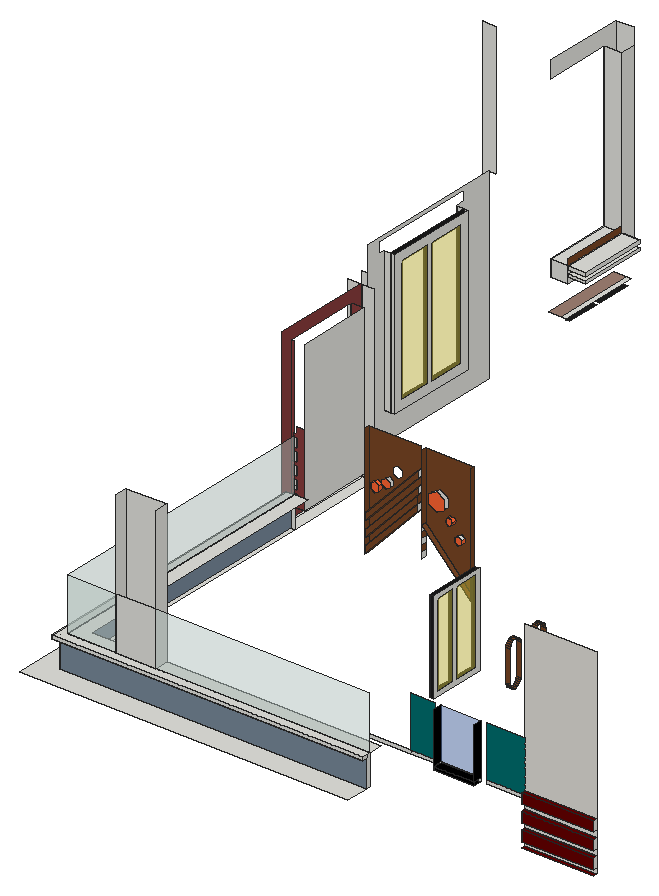
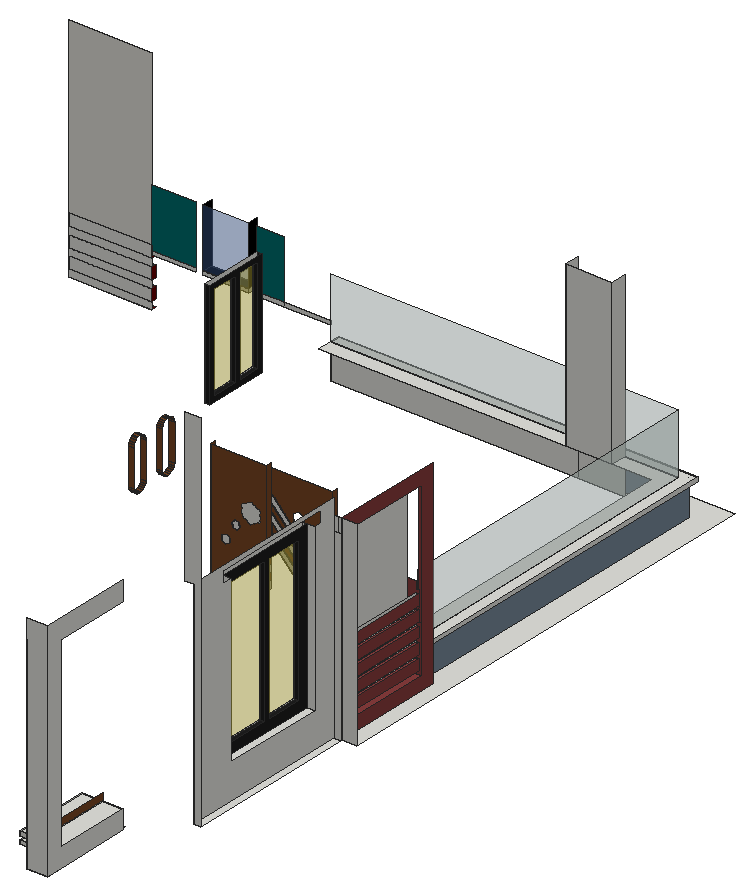
# SketchUp Ruby script. Lengths in inches.
U = 1.inch
M = Sketchup.active_model
def pt(a) = Geom::Point3d.new(a.map { |v| v * U })
def face(e, loops, mat)
  f = e.add_face(loops[0].map { |a| pt(a) })
  loops[1..].each { |l| e.add_face(l.map { |a| pt(a) }).erase! }
  f.material = f.back_material = mat if mat
  f
end
# faces: each face lists its corners as indices into pts; further lists are holes
def faces(e, pts, list, mat = nil) = list.each { |f| face(e, (f[0].is_a?(Array) ? f : [f]).map { |l| l.map { |i| pts[i] } }, mat) }
# xy, xz, yz: faces in a plane at the given z, y or x. An outline is a flat list of corners, or four numbers for a rectangle; further outlines are holes
def ring(l) = l.size == 4 ? [[l[0], l[1]], [l[2], l[1]], [l[2], l[3]], [l[0], l[3]]] : l.each_slice(2).to_a
def flat(e, list, mat, &to3) = list.each { |f| face(e, (f[0].is_a?(Array) ? f : [f]).map { |l| ring(l).map { |u, v| to3.(u, v) } }, mat) }
def xy(e, z, list, mat = nil) = flat(e, list, mat) { |x, y| [x, y, z] }
def xz(e, y, list, mat = nil) = flat(e, list, mat) { |x, z| [x, y, z] }
def yz(e, x, list, mat = nil) = flat(e, list, mat) { |y, z| [x, y, z] }
def lines(e, pts, list) = list.each { |a, b| e.add_line(pt(pts[a]), pt(pts[b])) }
# prism: a flat outline (further loops are holes) pulled along v
def prism(e, loops, v, mat = nil)
  f = face(e, loops, mat); d = Geom::Vector3d.new(v.map { |x| x * U })
  f.pushpull(f.normal.samedirection?(d) ? d.length : -d.length)
end
def box(e, o, s, mat = nil) = prism(e, [[o, [o[0] + s[0], o[1], o[2]], [o[0] + s[0], o[1] + s[1], o[2]], [o[0], o[1] + s[1], o[2]]]], [0, 0, s[2]], mat)
def at(x, y, z, deg = 0) = Geom::Transformation.translation(pt([x, y, z])) * Geom::Transformation.rotation(ORIGIN, Z_AXIS, deg.degrees)
def axes(o, x, y, z) = Geom::Transformation.new([*x, 0, *y, 0, *z, 0, *pt(o).to_a, 1])
def part(name) = M.definitions.add(name)
# library, detail: a bought-in or finely detailed component or shape, given as its bounding box
def library(name, o, s) = part(name).tap { |d| box(d.entities, o, s) }
def detail(e, o, s) = box(e.add_group.entities, o, s)
def put(e, d, t, mat = nil) = e.add_instance(d, t).tap { |i| i.material = mat if mat }
def group(e, t, mat = nil) = e.add_group.tap { |g| g.transformation = t; g.material = mat if mat }.entities
root = M.entities
M.materials.add("Niraj_Skin").color = [158, 128, 115]
M.materials.add("[0017_IndianRed]").color = [135, 60, 60]
M.materials.add("[0110_LightSlateGray]").color = [119, 136, 153]
M.materials.add("[Color A08]").color = [102, 0, 0]
M.materials.add("[Color B04]").color = [255, 101, 50]
M.materials.add("[Color H07]1").color = [0, 109, 109]
M.materials.add("[Color M08]").color = [30, 30, 30]
M.materials.add("[Color M09]").color = [0, 0, 0]
M.materials.add("[Marble Carrara Gold Floor Tile]").color = [225, 223, 217]
M.materials.add("[Translucent Glass Blue]").color = [218, 237, 231]
M.materials["[Translucent Glass Blue]"].alpha = 0.5
M.materials.add("[Translucent Glass Blue]1").color = [78, 117, 186]
M.materials["[Translucent Glass Blue]1"].alpha = 0.5
M.materials.add("[Translucent Glass Gray]").color = [242, 225, 74]
M.materials["[Translucent Glass Gray]"].alpha = 0.5
M.materials.add("[Wood Veneer 01]").color = [120, 70, 37]
xy(root,135.72,[[72.04,94.04,294.79,94.04,294.79,109.91,86.54,109.91,86.54,305.6,80.6,305.6,80.6,372.52,72.04,372.52],[86.54,109.91,121.875,112.91],[121.875,109.91,149.09,112.91],[149.09,109.91,294.79,112.91],[86.54,112.91,89.54,305.6],
  [80.6,305.6,82.23,372.52],[82.23,305.6,89.54,372.52]])
xy(root,136.63,[[400.27,109.91,449.03,112.91]],"[Color A08]")
xy(root,140.68,[[400.27,109.91,449.03,112.91]],"[Color A08]")
xy(root,143.24,[[72.04,383.99,76.23,487.33]])
xy(root,143.72,[[80.6,313.6,89.54,364.52]],"[0017_IndianRed]")
xy(root,145.85,[[82.23,313.6,84.23,364.52]],"[0017_IndianRed]")
xy(root,147.57,[[400.27,109.91,449.03,112.91]],"[Color A08]")
xy(root,152.12,[[82.23,313.6,84.23,364.52]],"[0017_IndianRed]")
xy(root,152.12,[[400.27,109.91,449.03,112.91]],"[Color A08]")
xy(root,154.35,[[83.54,106.91,83.54,305.6,86.54,305.6,86.54,109.91,294.79,109.91,294.79,106.91]])
xy(root,154.35,[[82.23,313.6,84.23,364.52]],"[0017_IndianRed]")
xy(root,156.61,[[83.54,106.91,294.79,106.91,294.79,112.91,89.54,112.91,89.54,305.6,83.54,305.6],[89.54,112.91,121.875,112.91,121.875,121.91,98.54,121.91,98.54,305.6,89.54,305.6],[121.875,112.91,149.09,121.91],[149.09,112.91,294.79,121.91]])
xy(root,159.01,[[400.27,109.91,449.03,112.91]],"[Color A08]")
xy(root,159.875,[[86.54,539.21,89.54,562],[86.54,565,89.54,588.21]],"[Color M08]")
xy(root,160.62,[[82.23,313.6,84.23,364.52]],"[0017_IndianRed]")
xy(root,162.85,[[82.23,313.6,84.23,364.52]],"[0017_IndianRed]")
xy(root,162.875,[[86.54,536.21,89.54,591.21]])
xy(root,162.875,[[77.54,536.21,86.54,591.21]],"Niraj_Skin")
xy(root,163.62,[[400.27,109.91,449.03,112.91]],"[Color A08]")
xy(root,163.625,[[76.23,397.54,81.04,459.54],[81.04,397.54,84.04,459.54]])
xy(root,165.31,[[291.79,167.29,294.79,205.98]])
xy(root,165.34,[[343.08,106.91,369.95,112.91]],"[Color M09]")
xy(root,167.72,[[343.08,106.91,369.95,112.91]],"[Color M09]")
xy(root,168.31,[[291.79,170.29,294.79,183.63],[291.79,186.63,294.79,202.98]],"[Color M08]")
xy(root,169.12,[[82.23,313.6,84.23,364.52]],"[0017_IndianRed]")
xy(root,169.625,[[81.04,403.54,84.04,425.54],[81.04,428.54,84.04,453.54]],"[Color M08]")
xy(root,170.51,[[400.27,109.91,449.03,112.91]],"[Color A08]")
xy(root,171.35,[[82.23,313.6,84.23,364.52]],"[0017_IndianRed]")
xy(root,172.4,[[65.54,552.74,77.54,608.18]])
xy(root,176.7,[[77.54,552.74,89.54,598.37]])
xy(root,177.62,[[82.23,313.6,84.23,364.52]],"[0017_IndianRed]")
xy(root,178.83,[[77.54,552.74,89.54,598.37]])
xy(root,179.85,[[82.23,313.6,84.23,364.52]],"[0017_IndianRed]")
xy(root,181.11,[[77.54,552.74,89.54,598.37]])
xy(root,183.52,[[65.54,552.74,77.54,598.37],[77.54,552.74,89.54,598.37]])
xz(root,106.91,[[83.54,154.35,294.79,156.61]])
xz(root,106.91,[[343.08,165.34,369.95,167.72]],"[Color M09]")
xz(root,109.91,[[86.54,135.72,294.79,154.35]],"[0110_LightSlateGray]")
xz(root,109.91,[[400.27,140.68,449.03,147.57],[400.27,152.12,449.03,159.01],[400.27,163.62,449.03,170.51]],"[Color A08]")
xz(root,112.91,[[121.875,135.72,149.09,156.61],[149.09,135.72,294.79,156.61],[400.27,136.63,449.03,140.68],[400.27,140.68,449.03,147.57],[400.27,147.57,449.03,152.12],
  [400.27,152.12,449.03,159.01],[121.875,156.61,149.09,192.65],[400.27,159.01,449.03,163.62],[400.27,163.62,449.03,170.51],[294.79,165.34,322.48,167.72],
  [322.48,165.34,338.5625,167.72],[343.08,165.34,369.95,167.72],[374.46,165.34,400.27,167.72]])
xz(root,112.91,[[322.48,167.72,338.5625,202.34],[374.46,167.72,400.27,202.34]],"[Color H07]1")
xz(root,112.91,[[400.27,170.51,449.03,272.06]],"[Marble Carrara Gold Floor Tile]")
xz(root,112.91,[[89.54,156.61,121.875,192.65],[149.09,156.61,294.79,192.65]],"[Translucent Glass Blue]")
xz(root,112.91,[[343.08,167.72,369.95,202.34]],"[Translucent Glass Blue]1")
xz(root,121.91,[[121.875,156.61,149.09,252.61]])
xz(root,167.29,[[291.79,165.31,294.79,227.91]],"[Color M08]")
xz(root,170.29,[[291.79,168.31,294.79,224.91]],"[Color M08]")
xz(root,183.63,[[291.79,168.31,294.79,224.91]],"[Color M08]")
xz(root,186.63,[[291.79,168.31,294.79,224.91]],"[Color M08]")
xz(root,202.98,[[291.79,168.31,294.79,224.91]],"[Color M08]")
xz(root,205.98,[[291.79,165.31,294.79,227.91]],"[Color M08]")
xz(root,231.95,[[291.79,145.88,294.79,167.68]],"[Wood Veneer 01]")
xz(root,240.95,[[291.79,145.88,294.79,167.68]],"[Wood Veneer 01]")
xz(root,252.89,[[291.79,145.55,294.79,167.31]],"[Wood Veneer 01]")
xz(root,261.89,[[291.79,145.55,294.79,167.31]],"[Wood Veneer 01]")
xz(root,302.6,[[202.79,166.82,205.12,168.17,205.12,170.85,202.79,172.2,200.46,170.85,200.46,168.17],[195.85,176.65,198.23,177.1875,198.95,179.52,197.29,181.31,194.92,180.76,194.2,178.44],[146.17,179.47,148.88,181.04,148.88,184.16,146.17,185.72,143.47,184.16,143.47,181.04],[188.08,182.05,193.38,185.11,193.38,191.23,188.08,194.3,182.77,191.23,182.77,185.11],[153.89,184.47,156.43,185.9375,156.43,188.875,153.89,190.34,151.34,188.875,151.34,185.9375]],"[Color B04]")
xz(root,302.6,[[139.47,139.77,175.47,178,175.47,182.94,139.47,144.71],[139.47,149.64,175.47,187.88,175.47,192.82,139.47,154.58],[139.47,159.52,175.47,197.75,175.47,202.69,139.47,164.46]],"[Wood Veneer 01]")
xz(root,305.6,[[86.54,135.72,89.54,156.61],[139.47,139.77,139.47,144.71,175.47,182.94,175.47,178],[139.47,149.64,139.47,154.58,175.47,192.82,175.47,187.88],[83.54,154.35,86.54,156.61],[139.47,159.52,139.47,164.46,175.47,202.69,175.47,197.75],
  [202.79,166.82,200.46,168.17,200.46,170.85,202.79,172.2,205.12,170.85,205.12,168.17],[195.85,176.65,194.2,178.44,194.92,180.76,197.29,181.31,198.95,179.52,198.23,177.1875],[146.17,179.47,143.47,181.04,143.47,184.16,146.17,185.72,148.88,184.16,148.88,181.04],[188.08,182.05,182.77,185.11,182.77,191.23,188.08,194.3,193.38,191.23,193.38,185.11],[153.89,184.47,151.34,185.9375,151.34,188.875,153.89,190.34,156.43,188.875,156.43,185.9375]])
xz(root,305.6,[[[211.47,136.41,211.47,216.61,178.47,216.61,178.47,171.19],[188.08,182.05,182.77,185.11,182.77,191.23,188.08,194.3,193.38,191.23,193.38,185.11],[202.79,166.82,200.46,168.17,200.46,170.85,202.79,172.2,205.12,170.85,205.12,168.17],[195.85,176.65,194.2,178.44,194.92,180.76,197.29,181.31,198.95,179.52,198.23,177.1875]],[139.47,144.71,175.47,182.94,175.47,187.88,139.47,149.64],[139.47,154.58,175.47,192.82,175.47,197.75,139.47,159.52],[[139.47,164.46,175.47,202.69,175.47,216.61,139.47,216.61],[159.61,191.2,156.25,193.13,156.25,197.01,159.61,198.95,162.97,197.01,162.97,193.13],[146.17,179.47,143.47,181.04,143.47,184.16,146.17,185.72,148.88,184.16,148.88,181.04],[153.89,184.47,151.34,185.9375,151.34,188.875,153.89,190.34,156.43,188.875,156.43,185.9375]]],"[Wood Veneer 01]")
xz(root,313.6,[[82.23,145.85,84.23,152.12],[82.23,154.35,84.23,156.61],[82.23,156.61,84.23,160.62],[82.23,162.85,84.23,169.12],[82.23,171.35,84.23,177.62],
  [82.23,179.85,84.23,186.12]])
xz(root,313.6,[[[80.6,143.72,80.6,171.35,84.23,171.35,84.23,177.62,82.23,177.62,82.23,179.85,84.23,179.85,84.23,186.12,82.23,186.12,82.23,188.35,84.23,188.35,84.23,192.65,89.54,192.65,89.54,156.61,84.23,156.61,84.23,160.62,82.23,160.62,82.23,154.35,84.23,154.35,84.23,156.61,89.54,156.61,89.54,143.72],[82.23,162.85,84.23,169.12],[82.23,145.85,84.23,152.12]],[80.6,171.35,82.23,244.62]],"[0017_IndianRed]")
xz(root,364.52,[[82.23,145.85,84.23,152.12],[82.23,154.35,84.23,160.62],[82.23,162.85,84.23,169.12],[82.23,171.35,84.23,177.62],[82.23,179.85,84.23,186.12]])
xz(root,364.52,[[80.6,143.72,89.54,143.72,89.54,244.62,82.23,244.62,82.23,237.12,84.23,237.12,84.23,230.85,82.23,230.85,82.23,228.62,84.23,228.62,84.23,222.35,82.23,222.35,82.23,220.12,84.23,220.12,84.23,213.85,82.23,213.85,82.23,211.62,84.23,211.62,84.23,205.35,82.23,205.35,82.23,203.12,84.23,203.12,84.23,196.85,82.23,196.85,82.23,194.62,84.23,194.62,84.23,188.35,82.23,188.35,82.23,186.12,84.23,186.12,84.23,179.85,82.23,179.85,82.23,177.62,84.23,177.62,84.23,171.35,82.23,171.35,82.23,169.12,84.23,169.12,84.23,162.85,82.23,162.85,82.23,160.62,84.23,160.62,84.23,154.35,82.23,154.35,82.23,152.12,84.23,152.12,84.23,145.85,82.23,145.85,82.23,244.62,80.6,244.62]],"[0017_IndianRed]")
xz(root,372.52,[[72.04,135.72,80.6,252.61],[80.6,135.72,82.23,252.61],[82.23,135.72,89.54,252.61]])
xz(root,383.99,[[72.04,143.24,76.23,252.61]])
xz(root,397.54,[[76.23,163.625,81.04,260.625],[81.04,163.625,84.04,260.5]])
xz(root,403.54,[[81.04,169.625,84.04,254.5]],"[Color M08]")
xz(root,425.54,[[81.04,169.625,84.04,254.5]],"[Color M08]")
xz(root,428.54,[[81.04,169.625,84.04,254.5]],"[Color M08]")
xz(root,453.54,[[81.04,169.625,84.04,254.5]],"[Color M08]")
xz(root,459.54,[[76.23,163.625,81.04,260.625],[81.04,163.625,84.04,260.5]])
xz(root,487.33,[[72.04,143.24,76.23,143.24,76.23,269.74,81.04,269.74,81.04,359.2,72.04,359.2]])
xz(root,552.74,[[65.54,172.4,77.54,183.52],[77.54,176.7,89.54,178.83],[77.54,181.11,89.54,183.52]])
xz(root,598.37,[[77.54,176.7,89.54,178.83],[77.54,181.11,89.54,183.52],[65.54,183.52,77.54,292.96]])
xz(root,608.18,[[65.54,172.4,77.54,304.46]])
yz(root,65.54,[[552.74,172.4,552.74,183.52,598.37,183.52,598.37,292.96,552.74,292.96,552.74,304.46,608.18,304.46,608.18,172.4]])
yz(root,76.23,[[[383.99,143.24,487.33,269.74],[397.54,163.625,459.54,163.625,459.54,260.625,465.79,260.625,465.79,267.49,393.2,267.49,393.2,260.625,397.54,260.625]]])
yz(root,77.54,[[552.74,172.4,552.74,176.7,598.37,176.7,598.37,178.83,552.74,178.83,552.74,181.11,598.37,181.11,598.37,292.96,608.18,292.96,608.18,172.4],[552.74,176.7,598.37,178.83],[552.74,181.11,598.37,183.52]])
yz(root,77.54,[[552.74,183.52,598.37,187.92]],"[Wood Veneer 01]")
yz(root,80.6,[[[305.6,135.72,372.52,252.61],[313.6,143.72,364.52,244.62]]],"[0017_IndianRed]")
yz(root,81.04,[[[397.54,163.625,459.54,260.5],[428.54,169.625,453.54,254.5],[403.54,169.625,425.54,254.5]]],"[Color M08]")
yz(root,82.23,[[313.6,145.85,364.52,152.12],[313.6,154.35,364.52,160.62],[313.6,162.85,364.52,169.12],[313.6,171.35,364.52,177.62],[313.6,179.85,364.52,186.12]],"[0017_IndianRed]")
yz(root,83.54,[[106.91,154.35,305.6,156.61]])
yz(root,84.04,[[[397.54,163.625,459.54,260.5],[428.54,169.625,453.54,254.5],[403.54,169.625,425.54,254.5]]])
yz(root,84.04,[[403.54,169.625,425.54,254.5],[428.54,169.625,453.54,254.5]],"[Translucent Glass Gray]")
yz(root,84.23,[[313.6,145.85,364.52,152.12],[313.6,154.35,364.52,160.62],[313.6,162.85,364.52,169.12],[313.6,171.35,364.52,177.62],[313.6,179.85,364.52,186.12]])
yz(root,86.54,[[109.91,135.72,305.6,154.35]],"[0110_LightSlateGray]")
yz(root,89.54,[[313.6,143.72,364.52,244.62],[552.74,176.7,598.37,178.83],[552.74,181.11,598.37,183.52]])
yz(root,89.54,[[112.91,156.61,305.6,192.65]],"[Translucent Glass Blue]")
yz(root,121.875,[[112.91,156.61,121.91,252.61]])
yz(root,139.47,[[302.6,139.77,305.6,144.71],[302.6,149.64,305.6,154.58],[302.6,159.52,305.6,164.46]])
yz(root,139.47,[[302.6,144.71,305.6,149.64],[302.6,154.58,305.6,159.52],[302.6,164.46,305.6,216.61]],"[Wood Veneer 01]")
yz(root,143.47,[[302.6,181.04,305.6,184.16]],"[Color B04]")
yz(root,148.88,[[302.6,181.04,305.6,184.16]],"[Color B04]")
yz(root,149.09,[[112.91,156.61,121.91,252.61]])
yz(root,175.47,[[302.6,178,305.6,182.94]])
yz(root,175.47,[[302.6,182.94,305.6,187.88]],"[Wood Veneer 01]")
yz(root,178.47,[[302.6,150.57,305.6,154.69],[302.6,158.82,305.6,162.94],[302.6,167.07,305.6,171.19]])
yz(root,178.47,[[302.6,154.69,305.6,158.82],[302.6,162.94,305.6,167.07],[302.6,171.19,305.6,216.61]],"[Wood Veneer 01]")
yz(root,200.46,[[302.6,168.17,305.6,170.85]],"[Color B04]")
yz(root,205.12,[[302.6,168.17,305.6,170.85]],"[Color B04]")
yz(root,211.47,[[302.6,136.41,305.6,216.61]],"[Wood Veneer 01]")
yz(root,291.79,[[[167.29,165.31,205.98,227.91],[186.63,168.31,202.98,224.91],[170.29,168.31,183.63,224.91]]],"[Color M08]")
yz(root,294.79,[[109.91,135.72,112.91,156.61],[106.91,154.35,109.91,156.61],[[167.29,165.31,205.98,227.91],[186.63,168.31,202.98,224.91],[170.29,168.31,183.63,224.91]]])
yz(root,294.79,[[170.29,168.31,183.63,224.91],[186.63,168.31,202.98,224.91]],"[Translucent Glass Gray]")
yz(root,343.08,[[106.91,165.34,112.91,167.72]])
yz(root,343.08,[[106.91,167.72,112.91,202.34]],"[Color M09]")
yz(root,369.95,[[106.91,167.72,112.91,202.34]],"[Color M09]")
yz(root,400.27,[[109.91,170.29,112.91,170.51]])
yz(root,400.27,[[109.91,140.68,112.91,147.57],[109.91,152.12,112.91,159.01],[109.91,163.62,112.91,170.29]],"[Color A08]")
yz(root,449.03,[[109.91,140.68,112.91,147.57],[109.91,152.12,112.91,159.01],[109.91,163.62,112.91,170.51]])
p = [[211.47,305.6,136.41],[178.47,305.6,171.19],[178.47,302.6,171.19],[211.47,302.6,136.41],[139.47,305.6,139.77],[175.47,305.6,178],
  [175.47,302.6,178],[139.47,302.6,139.77],[291.79,257.39,141.35],[291.79,256.27,141.49],[294.79,256.27,141.49],[294.79,257.39,141.35],
  [291.79,258.51,141.49],[294.79,258.51,141.49],[291.79,236.45,141.38],[291.79,235.29,141.54],[294.79,235.29,141.54],[294.79,236.45,141.38],
  [291.79,237.62,141.54],[294.79,237.62,141.54],[291.79,234.2,141.99],[294.79,234.2,141.99],[291.79,238.7,141.99],[294.79,238.7,141.99],
  [291.79,255.22,141.9],[294.79,255.22,141.9],[291.79,259.56,141.9],[294.79,259.56,141.9],[291.79,254.3125,142.5625],[294.79,254.3125,142.5625],
  [291.79,260.47,142.5625],[294.79,260.47,142.5625],[291.79,233.27,142.7],[294.79,233.27,142.7],[291.79,239.63,142.7],[294.79,239.63,142.7],
  [291.79,253.59,143.43],[294.79,253.59,143.43],[291.79,261.19,143.43],[294.79,261.19,143.43],[291.79,232.56,143.63],[294.79,232.56,143.63],
  [291.79,240.35,143.63],[294.79,240.35,143.63],[291.79,253.11,144.45],[294.79,253.11,144.45],[291.79,261.67,144.45],[294.79,261.67,144.45],
  [291.79,232.11,144.72],[294.79,232.11,144.72],[291.79,240.8,144.72],[294.79,240.8,144.72],[291.79,252.89,145.55],[294.79,252.89,145.55],
  [291.79,261.89,145.55],[294.79,261.89,145.55],[291.79,231.95,145.88],[294.79,231.95,145.88],[291.79,240.95,145.88],[294.79,240.95,145.88],
  [175.47,305.6,182.94],[139.47,305.6,144.71],[139.47,302.6,144.71],[175.47,302.6,182.94],[139.47,305.6,149.64],[175.47,305.6,187.88],
  [175.47,302.6,187.88],[139.47,302.6,149.64],[175.47,305.6,192.82],[139.47,305.6,154.58],[139.47,302.6,154.58],[175.47,302.6,192.82],
  [139.47,305.6,159.52],[175.47,305.6,197.75],[175.47,302.6,197.75],[139.47,302.6,159.52],[175.47,305.6,202.69],[139.47,305.6,164.46],
  [139.47,302.6,164.46],[175.47,302.6,202.69],[200.46,305.6,168.17],[202.79,305.6,166.82],[202.79,302.6,166.82],[200.46,302.6,168.17],
  [205.12,305.6,168.17],[205.12,302.6,168.17],[291.79,252.89,167.31],[291.79,253.04,168.47],[294.79,253.04,168.47],[294.79,252.89,167.31],
  [291.79,261.74,168.47],[291.79,261.89,167.31],[294.79,261.89,167.31],[294.79,261.74,168.47],[291.79,231.95,167.68],[291.79,232.18,168.78],
  [294.79,232.18,168.78],[294.79,231.95,167.68],[291.79,240.73,168.78],[291.79,240.95,167.68],[294.79,240.95,167.68],[294.79,240.73,168.78],
  [291.79,253.49,169.56],[294.79,253.49,169.56],[291.79,261.29,169.56],[294.79,261.29,169.56],[291.79,232.66,169.79],[294.79,232.66,169.79],
  [291.79,240.24,169.79],[294.79,240.24,169.79],[291.79,254.21,170.49],[294.79,254.21,170.49],[291.79,260.57,170.49],[294.79,260.57,170.49],
  [291.79,233.39,170.65],[294.79,233.39,170.65],[291.79,239.52,170.65],[294.79,239.52,170.65],[291.79,255.14,171.21],[294.79,255.14,171.21],
  [291.79,259.64,171.21],[294.79,259.64,171.21],[291.79,234.3,171.3],[294.79,234.3,171.3],[291.79,238.61,171.3],[294.79,238.61,171.3],
  [202.79,305.6,172.2],[200.46,305.6,170.85],[200.46,302.6,170.85],[202.79,302.6,172.2],[205.12,305.6,170.85],[205.12,302.6,170.85],
  [291.79,256.23,171.65],[294.79,256.23,171.65],[291.79,258.55,171.65],[294.79,258.55,171.65],[291.79,235.34,171.71],[294.79,235.34,171.71],
  [291.79,237.57,171.71],[294.79,237.57,171.71],[291.79,236.45,171.85],[294.79,236.45,171.85],[291.79,257.39,171.81],[294.79,257.39,171.81],
  [194.2,305.6,178.44],[195.85,305.6,176.65],[195.85,302.6,176.65],[194.2,302.6,178.44],[198.23,305.6,177.1875],[198.23,302.6,177.1875],
  [198.95,305.6,179.52],[198.95,302.6,179.52],[194.92,305.6,180.76],[194.92,302.6,180.76],[143.47,305.6,181.04],[146.17,305.6,179.47],
  [146.17,302.6,179.47],[143.47,302.6,181.04],[148.88,305.6,181.04],[148.88,302.6,181.04],[197.29,305.6,181.31],[197.29,302.6,181.31],
  [182.77,305.6,185.11],[188.08,305.6,182.05],[188.08,302.6,182.05],[182.77,302.6,185.11],[193.38,305.6,185.11],[193.38,302.6,185.11],
  [146.17,305.6,185.72],[143.47,305.6,184.16],[143.47,302.6,184.16],[146.17,302.6,185.72],[148.88,305.6,184.16],[148.88,302.6,184.16],
  [151.34,305.6,185.9375],[153.89,305.6,184.47],[153.89,302.6,184.47],[151.34,302.6,185.9375],[156.43,305.6,185.9375],[156.43,302.6,185.9375],
  [86.54,109.91,154.35],[86.54,109.91,156.61]]
faces(root,p,[[0,1,2,3],[4,5,6,7],[8,9,10,11],[12,8,11,13],[14,15,16,17],[18,14,17,19],[15,20,21,16],[22,18,19,23],
  [9,24,25,10],[26,12,13,27],[24,28,29,25],[30,26,27,31],[20,32,33,21],[34,22,23,35],[28,36,37,29],[38,30,31,39],
  [32,40,41,33],[42,34,35,43],[36,44,45,37],[46,38,39,47],[40,48,49,41],[50,42,43,51],[44,52,53,45],[54,46,47,55],
  [48,56,57,49],[58,50,51,59],[60,61,62,63],[64,65,66,67],[68,69,70,71],[72,73,74,75],[76,77,78,79],[86,87,88,89],
  [90,91,92,93],[94,95,96,97],[98,99,100,101],[87,102,103,88],[104,90,93,105],[95,106,107,96],[108,98,101,109],[102,110,111,103],
  [112,104,105,113],[106,114,115,107],[116,108,109,117],[110,118,119,111],[120,112,113,121],[114,122,123,115],[124,116,117,125],[118,132,133,119],
  [134,120,121,135],[122,136,137,123],[138,124,125,139],[136,140,141,137],[140,138,139,141],[132,142,143,133],[142,134,135,143]],"[Wood Veneer 01]")
faces(root,p,[[80,81,82,83],[81,84,85,82],[126,127,128,129],[144,145,146,147],[145,148,149,146],[148,150,151,149],[152,144,147,153],[154,155,156,157],
  [155,158,159,156],[150,160,161,151],[160,152,153,161],[162,163,164,165],[163,166,167,164],[168,169,170,171],[172,168,171,173],[174,175,176,177],
  [175,178,179,176]],"[Color B04]")
faces(root,p,[[130,126,129,131]])
lines(root,p,[[180,181]])
